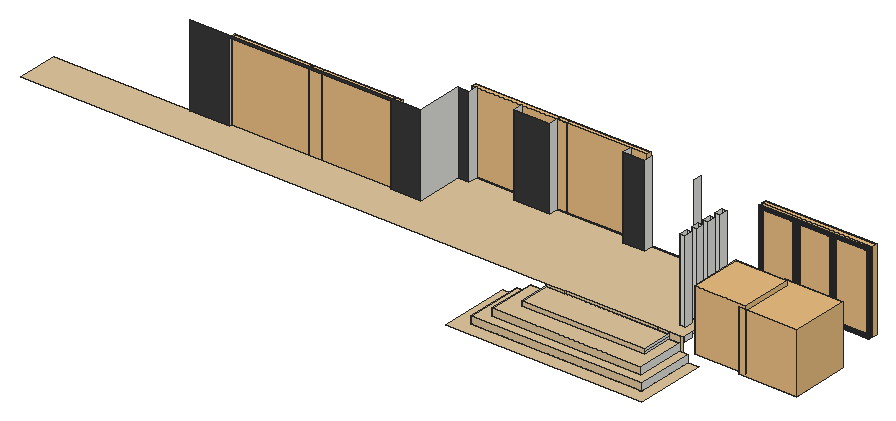
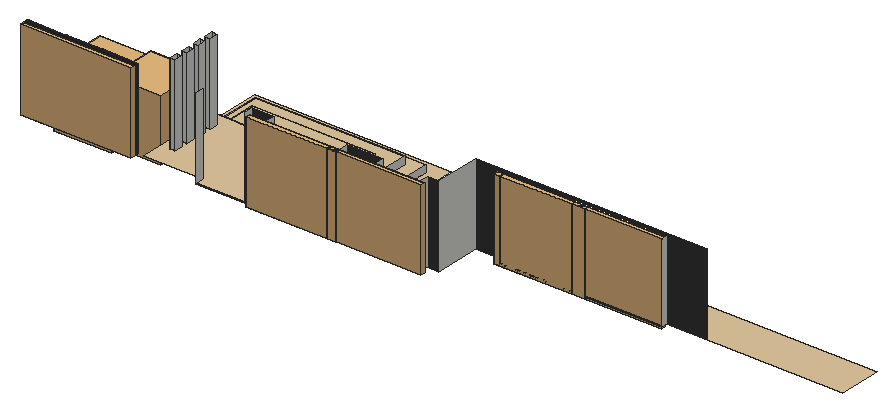
# SketchUp Ruby script. Lengths in inches.
U = 1.inch
M = Sketchup.active_model
def pt(a) = Geom::Point3d.new(a.map { |v| v * U })
def face(e, loops, mat)
  f = e.add_face(loops[0].map { |a| pt(a) })
  loops[1..].each { |l| e.add_face(l.map { |a| pt(a) }).erase! }
  f.material = f.back_material = mat if mat
  f
end
# faces: each face lists its corners as indices into pts; further lists are holes
def faces(e, pts, list, mat = nil) = list.each { |f| face(e, (f[0].is_a?(Array) ? f : [f]).map { |l| l.map { |i| pts[i] } }, mat) }
# xy, xz, yz: faces in a plane at the given z, y or x. An outline is a flat list of corners, or four numbers for a rectangle; further outlines are holes
def ring(l) = l.size == 4 ? [[l[0], l[1]], [l[2], l[1]], [l[2], l[3]], [l[0], l[3]]] : l.each_slice(2).to_a
def flat(e, list, mat, &to3) = list.each { |f| face(e, (f[0].is_a?(Array) ? f : [f]).map { |l| ring(l).map { |u, v| to3.(u, v) } }, mat) }
def xy(e, z, list, mat = nil) = flat(e, list, mat) { |x, y| [x, y, z] }
def xz(e, y, list, mat = nil) = flat(e, list, mat) { |x, z| [x, y, z] }
def yz(e, x, list, mat = nil) = flat(e, list, mat) { |y, z| [x, y, z] }
def lines(e, pts, list) = list.each { |a, b| e.add_line(pt(pts[a]), pt(pts[b])) }
# prism: a flat outline (further loops are holes) pulled along v
def prism(e, loops, v, mat = nil)
  f = face(e, loops, mat); d = Geom::Vector3d.new(v.map { |x| x * U })
  f.pushpull(f.normal.samedirection?(d) ? d.length : -d.length)
end
def box(e, o, s, mat = nil) = prism(e, [[o, [o[0] + s[0], o[1], o[2]], [o[0] + s[0], o[1] + s[1], o[2]], [o[0], o[1] + s[1], o[2]]]], [0, 0, s[2]], mat)
def at(x, y, z, deg = 0) = Geom::Transformation.translation(pt([x, y, z])) * Geom::Transformation.rotation(ORIGIN, Z_AXIS, deg.degrees)
def axes(o, x, y, z) = Geom::Transformation.new([*x, 0, *y, 0, *z, 0, *pt(o).to_a, 1])
def part(name) = M.definitions.add(name)
# library, detail: a bought-in or finely detailed component or shape, given as its bounding box
def library(name, o, s) = part(name).tap { |d| box(d.entities, o, s) }
def detail(e, o, s) = box(e.add_group.entities, o, s)
def put(e, d, t, mat = nil) = e.add_instance(d, t).tap { |i| i.material = mat if mat }
def group(e, t, mat = nil) = e.add_group.tap { |g| g.transformation = t; g.material = mat if mat }.entities
root = M.entities
M.materials.add("Wine2").color = [0, 0, 0]
M.materials["Wine2"].alpha = 0
M.materials.add("[0130_Gainsboro]").color = [39, 45, 50]
M.materials.add("[Color M08]").color = [56, 56, 56]
M.materials.add("[Formica Beige]").color = [226, 199, 158]
c1 = library("Plant+++Pot",[-21.48,-119.36,-205.6875],[86.44,86.43,89.41])
c2 = library("Floor plant",[-5.56,-16.3125,0.81],[76.88,76.71,92.33])
c3 = library("Group5_1",[-7.56,-66.38,0.11],[6.33,135.04,120.95])
c4 = part("Framed glazing panel")
xy(c4.entities,0,[[0,-0.98,43.07,0],[0,0,43.07,1.4]],"[0130_Gainsboro]")
xy(c4.entities,0.3,[[0.3,-1.43,42.77,-0.98]],"[0130_Gainsboro]")
xy(c4.entities,2.95,[[2.95,-1.43,40.12,-0.63],[2.95,-0.63,40.12,0],[2.95,0,40.12,0.64],[2.95,0.64,40.12,1.4]],"[0130_Gainsboro]")
xy(c4.entities,3.54,[[3.54,-0.63,39.53,0],[3.54,0,39.53,0.64]],"[0130_Gainsboro]")
xy(c4.entities,111.8125,[[3.54,-0.63,39.53,0],[3.54,0,39.53,0.64]],"[0130_Gainsboro]")
xy(c4.entities,112.4,[[2.95,-1.43,40.12,-0.63],[2.95,-0.63,40.12,0],[2.95,0,40.12,0.64],[2.95,0.64,40.12,1.4]],"[0130_Gainsboro]")
xy(c4.entities,115.05,[[0.3,-1.43,42.77,-0.98]],"[0130_Gainsboro]")
xy(c4.entities,115.35,[[0,-0.98,43.07,0],[0,0,43.07,1.4]],"[0130_Gainsboro]")
xz(c4.entities,-1.43,[[[0.3,0.3,42.77,115.05],[2.95,2.95,40.12,112.4]]],"[0130_Gainsboro]")
xz(c4.entities,-0.98,[[[0,0,43.07,115.35],[0.3,0.3,42.77,115.05]]],"[0130_Gainsboro]")
xz(c4.entities,-0.63,[[[2.95,2.95,40.12,112.4],[3.54,3.54,39.53,111.8125]]],"[0130_Gainsboro]")
xz(c4.entities,0,[[3.54,3.54,39.53,111.8125]],"Wine2")
xz(c4.entities,0,[[[0,0,43.07,115.35],[2.95,2.95,40.12,112.4]],[[2.95,2.95,40.12,112.4],[3.54,3.54,39.53,111.8125]]],"[0130_Gainsboro]")
xz(c4.entities,0.64,[[[2.95,2.95,40.12,112.4],[3.54,3.54,39.53,111.8125]]],"[0130_Gainsboro]")
xz(c4.entities,1.4,[[[0,0,43.07,115.35],[2.95,2.95,40.12,112.4]]],"[0130_Gainsboro]")
yz(c4.entities,0,[[-0.98,0,0,115.35],[0,0,1.4,115.35]],"[0130_Gainsboro]")
yz(c4.entities,0.3,[[-1.43,0.3,-0.98,115.05]],"[0130_Gainsboro]")
yz(c4.entities,2.95,[[-1.43,2.95,-0.63,112.4],[-0.63,2.95,0,112.4],[0,2.95,0.64,112.4],[0.64,2.95,1.4,112.4]],"[0130_Gainsboro]")
yz(c4.entities,3.54,[[-0.63,3.54,0,111.8125],[0,3.54,0.64,111.8125]],"[0130_Gainsboro]")
yz(c4.entities,39.53,[[-0.63,3.54,0,111.8125],[0,3.54,0.64,111.8125]],"[0130_Gainsboro]")
yz(c4.entities,40.12,[[-1.43,2.95,-0.63,112.4],[-0.63,2.95,0,112.4],[0,2.95,0.64,112.4],[0.64,2.95,1.4,112.4]],"[0130_Gainsboro]")
yz(c4.entities,42.77,[[-1.43,0.3,-0.98,115.05]],"[0130_Gainsboro]")
yz(c4.entities,43.07,[[-0.98,0,0,115.35],[0,0,1.4,115.35]],"[0130_Gainsboro]")
c5 = part("Glazed screen")
put(c5.entities,c4,axes([90.57,1.43,0],[1.05148,0,0],[0,1,0],[0,0,1]))
put(c5.entities,c4,axes([0,1.43,0],[1.05148,0,0],[0,1,0],[0,0,1]))
put(c5.entities,c4,axes([45.29,1.43,0],[1.05148,0,0],[0,1,0],[0,0,1]))
xy(root,18.94,[[722.74,167.6875,1015.74,167.6875,1015.74,274.5,1000.23,274.5,1000.23,187.3125,744.1,187.3125,744.1,274.5,722.74,274.5],[744.1,187.3125,1000.23,274.5]],"[Formica Beige]")
xy(root,19.02,[[744.1,187.3125,1000.23,274.5],[815.6,274.5,954.29,275.375]])
xy(root,29.9,[[815.6,274.5,954.29,275.375]])
xy(root,29.9,[[744.1,187.3125,1000.23,187.3125,1000.23,274.5,987.01,274.5,987.01,202.9375,763.95,202.9375,763.95,274.5,744.1,274.5],[763.95,202.9375,987.01,274.5]],"[Formica Beige]")
xy(root,40.875,[[763.95,202.9375,987.01,202.9375,987.01,274.5,971.35,274.5,971.35,228.5,787.73,228.5,787.73,274.5,763.95,274.5]],"[Formica Beige]")
xy(root,47.125,[[787.73,228.5,971.35,274.5]],"[Formica Beige]")
xy(root,50.65,[[0,274.5,815.6,274.5,815.6,275.375,954.29,275.375,954.29,274.5,991.92,274.5,991.92,406.8125,903,406.8125,903,420.5625,828.83,420.5625,828.83,406.8125,797.18,406.8125,797.18,420.5625,687.15,420.5625,687.15,406.8125,633.8,406.8125,633.8,420.5625,566.51,420.5625,566.51,406.8125,549.32,406.8125,549.32,336.9375,504.95,336.9375,504.95,347.22,263.51,347.22,263.51,336.9375,0,336.9375]],"[Formica Beige]")
xz(root,187.3125,[[744.1,18.94,1000.23,19.02],[744.1,19.02,1000.23,29.9]],"[Formica Beige]")
xz(root,202.9375,[[763.95,29.9,987.01,40.875]],"[Formica Beige]")
xz(root,228.5,[[787.73,40.875,971.35,47.125]],"[Formica Beige]")
xz(root,274.5,[[991.92,18.94,1000.23,19.02],[744.1,19.02,815.6,29.9],[815.6,19.02,954.29,29.9],[954.29,19.02,991.92,29.9],[763.95,29.9,787.73,40.875],
  [787.73,29.9,815.6,43.5625],[815.6,29.9,954.29,43.5625],[954.29,29.9,971.35,43.5625],[971.35,29.9,987.01,40.875],[787.73,43.5625,815.6,47.125],
  [815.6,43.5625,954.29,47.125],[954.29,43.5625,971.35,47.125]])
xz(root,274.5,[[744.1,18.94,991.92,19.02],[991.92,19.02,1000.23,29.9],[987.01,29.9,991.92,50.65],[971.35,40.875,987.01,50.65],[787.73,47.125,815.6,50.65],
  [954.29,47.125,971.35,50.65]],"[Formica Beige]")
xz(root,275.375,[[815.6,19.02,954.29,29.9]])
xz(root,275.375,[[815.6,29.9,954.29,50.65]],"[Formica Beige]")
xz(root,295.36,[[971.33,29.9,979.08,172.0625]])
xz(root,307.9,[[971.33,29.9,979.08,172.0625]])
xz(root,316.67,[[971.33,29.9,979.08,172.0625]])
xz(root,329.21,[[971.33,29.9,979.08,172.0625]])
xz(root,336.9375,[[204.29,50.65,263.51,50.65,263.51,168.9375,504.95,168.9375,504.95,50.65,549.32,50.65,549.32,172.0625,204.29,172.0625]],"[Color M08]")
xz(root,338.36,[[971.33,29.9,979.08,172.0625]])
xz(root,347.22,[[263.51,50.65,504.95,52.0625]])
xz(root,350.9,[[971.33,29.9,979.08,172.0625]])
xz(root,360.8,[[971.33,29.9,979.08,172.0625]])
xz(root,373.34,[[971.33,29.9,979.08,172.0625]])
xz(root,406.8125,[[549.32,50.65,566.51,172.0625],[633.8,50.65,687.15,172.0625],[797.18,50.65,828.83,172.0625]],"[Color M08]")
xz(root,420.5625,[[566.51,50.65,633.8,52.0625],[687.15,50.65,797.18,52.0625],[828.83,50.65,903,52.0625]])
yz(root,263.51,[[336.9375,50.65,347.22,168.9375]])
yz(root,504.95,[[336.9375,50.65,347.22,168.9375]])
yz(root,549.32,[[336.9375,50.65,406.8125,172.0625]])
yz(root,566.51,[[406.8125,50.65,420.5625,172.0625]])
yz(root,633.8,[[406.8125,50.65,420.5625,172.0625]])
yz(root,687.15,[[406.8125,50.65,420.5625,172.0625]])
yz(root,744.1,[[187.3125,19.02,274.5,29.9]])
yz(root,744.1,[[187.3125,18.94,274.5,19.02]],"[Formica Beige]")
yz(root,763.95,[[202.9375,29.9,274.5,40.875]])
yz(root,787.73,[[228.5,40.875,274.5,47.125]])
yz(root,797.18,[[406.8125,50.65,420.5625,172.0625]])
yz(root,815.6,[[274.5,19.02,275.375,29.9]])
yz(root,815.6,[[274.5,29.9,275.375,50.65]],"[Formica Beige]")
yz(root,828.83,[[406.8125,50.65,420.5625,172.0625]])
yz(root,903,[[406.8125,50.65,420.5625,172.0625]])
yz(root,954.29,[[274.5,19.02,275.375,29.9]])
yz(root,954.29,[[274.5,29.9,275.375,50.65]],"[Formica Beige]")
yz(root,971.33,[[295.36,29.9,307.9,172.0625],[316.67,29.9,329.21,172.0625],[338.36,29.9,350.9,172.0625],[360.8,29.9,373.34,172.0625]])
yz(root,971.35,[[228.5,40.875,274.5,43.5625],[228.5,43.5625,274.5,47.125]])
yz(root,979.08,[[295.36,29.9,307.9,172.0625],[316.67,29.9,329.21,172.0625],[338.36,29.9,350.9,172.0625],[360.8,29.9,373.34,172.0625]])
yz(root,987.01,[[202.9375,29.9,274.5,40.875]])
yz(root,1000.23,[[187.3125,19.02,274.5,29.9]])
yz(root,1000.23,[[187.3125,18.94,274.5,19.02]],"[Formica Beige]")
put(root,c1,at(1082.77,412.09,223.38))
put(root,c2,at(1001.1,309.05,19.99))
put(root,c3,at(445.39,339.66,47.88,-90))
put(root,c3,at(329.89,339.66,47.88,-90))
put(root,c5,axes([999.71,406.36,51.09],[1.221,0,0],[0,1,0],[0,0,1.04867]))
put(root,c3,at(753.52,419.34,51,-90))
put(root,c3,axes([629.45,419.34,51],[0,-1,0],[1.05,0,0],[0,0,1]))
put(root,c3,axes([1081.2,412.46,51],[0,-1,0],[1.22916,0,0],[0,0,1]))
